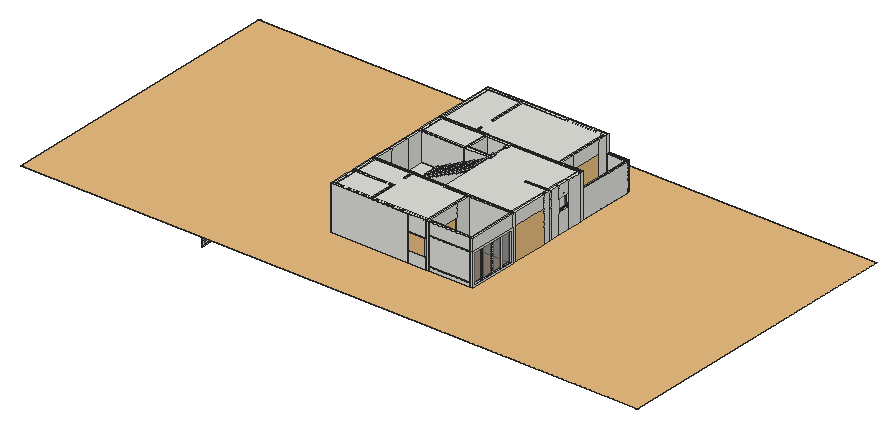
# SketchUp Ruby script. Lengths in inches.
U = 1.inch
M = Sketchup.active_model
def pt(a) = Geom::Point3d.new(a.map { |v| v * U })
def face(e, loops, mat)
  f = e.add_face(loops[0].map { |a| pt(a) })
  loops[1..].each { |l| e.add_face(l.map { |a| pt(a) }).erase! }
  f.material = f.back_material = mat if mat
  f
end
# faces: each face lists its corners as indices into pts; further lists are holes
def faces(e, pts, list, mat = nil) = list.each { |f| face(e, (f[0].is_a?(Array) ? f : [f]).map { |l| l.map { |i| pts[i] } }, mat) }
# xy, xz, yz: faces in a plane at the given z, y or x. An outline is a flat list of corners, or four numbers for a rectangle; further outlines are holes
def ring(l) = l.size == 4 ? [[l[0], l[1]], [l[2], l[1]], [l[2], l[3]], [l[0], l[3]]] : l.each_slice(2).to_a
def flat(e, list, mat, &to3) = list.each { |f| face(e, (f[0].is_a?(Array) ? f : [f]).map { |l| ring(l).map { |u, v| to3.(u, v) } }, mat) }
def xy(e, z, list, mat = nil) = flat(e, list, mat) { |x, y| [x, y, z] }
def xz(e, y, list, mat = nil) = flat(e, list, mat) { |x, z| [x, y, z] }
def yz(e, x, list, mat = nil) = flat(e, list, mat) { |y, z| [x, y, z] }
def lines(e, pts, list) = list.each { |a, b| e.add_line(pt(pts[a]), pt(pts[b])) }
# prism: a flat outline (further loops are holes) pulled along v
def prism(e, loops, v, mat = nil)
  f = face(e, loops, mat); d = Geom::Vector3d.new(v.map { |x| x * U })
  f.pushpull(f.normal.samedirection?(d) ? d.length : -d.length)
end
def box(e, o, s, mat = nil) = prism(e, [[o, [o[0] + s[0], o[1], o[2]], [o[0] + s[0], o[1] + s[1], o[2]], [o[0], o[1] + s[1], o[2]]]], [0, 0, s[2]], mat)
def at(x, y, z, deg = 0) = Geom::Transformation.translation(pt([x, y, z])) * Geom::Transformation.rotation(ORIGIN, Z_AXIS, deg.degrees)
def axes(o, x, y, z) = Geom::Transformation.new([*x, 0, *y, 0, *z, 0, *pt(o).to_a, 1])
def part(name) = M.definitions.add(name)
# library, detail: a bought-in or finely detailed component or shape, given as its bounding box
def library(name, o, s) = part(name).tap { |d| box(d.entities, o, s) }
def detail(e, o, s) = box(e.add_group.entities, o, s)
def put(e, d, t, mat = nil) = e.add_instance(d, t).tap { |i| i.material = mat if mat }
def group(e, t, mat = nil) = e.add_group.tap { |g| g.transformation = t; g.material = mat if mat }.entities
root = M.entities
M.materials.add("BeigeGloss_500x700").color = [214, 201, 185]
M.materials.add("MADEIRAS PORTAS MOD 4").color = [48, 37, 30]
M.materials.add("Metal_07").color = [114, 116, 119]
M.materials.add("Metal_Aluminum_Anodized").color = [200, 209, 218]
M.materials.add("Translucent_Glass_Gray").color = [198, 198, 198]
M.materials["Translucent_Glass_Gray"].alpha = 0.2
M.materials.add("[0136_Charcoal]1").color = [35, 35, 35]
M.materials.add("[Color_008]2").color = [30, 30, 30]
M.materials.add("[Translucent Glass Gray]").color = [128, 128, 128]
M.materials["[Translucent Glass Gray]"].alpha = 0.5
M.materials.add("[Translucent_Glass_Gray]").color = [128, 128, 128]
M.materials["[Translucent_Glass_Gray]"].alpha = 0.5
M.materials.add("aidan_hegarty_redux").color = [127, 127, 127]
M.materials["aidan_hegarty_redux"].alpha = 0
M.materials.add("door-silver").color = [161, 152, 147]
M.materials.add("wood _table").color = [169, 145, 123]
c1 = library("EAST VILLa 27.dwg",[0,0,0],[1841.08,888.15,0.01])
c2 = part("Untitled (3)")
g1 = group(c2.entities,at(-587.35,0.56,0))
g2 = group(g1,at(0,36.17,0))
g3 = group(g2,at(0,0,0))
xy(g3,0,[[0,-36.17,1118.43,-19.76]],"BeigeGloss_500x700")
xy(g3,7.07,[[6.51,-36.17,1111.93,-19.76]],"BeigeGloss_500x700")
xy(g3,448.65,[[6.51,-36.17,1111.93,-19.76]],"BeigeGloss_500x700")
xy(g3,455.72,[[0,-36.17,1118.43,-19.76]],"BeigeGloss_500x700")
xz(g3,-36.17,[[6.51,7.07,1111.93,448.65]])
xz(g3,-36.17,[[[0,0,1118.43,455.72],[6.51,7.07,1111.93,448.65]]],"BeigeGloss_500x700")
xz(g3,-19.76,[[[0,0,1118.43,455.72],[6.51,7.07,1111.93,448.65]]],"BeigeGloss_500x700")
yz(g3,0,[[-36.17,0,-19.76,455.72]],"BeigeGloss_500x700")
yz(g3,6.51,[[-36.17,7.07,-19.76,448.65]],"BeigeGloss_500x700")
yz(g3,1111.93,[[-36.17,7.07,-19.76,448.65]],"BeigeGloss_500x700")
yz(g3,1118.43,[[-36.17,0,-19.76,455.72]],"BeigeGloss_500x700")
c3 = part("Group\#69")
p = [[0,43.31,5.11],[2.95,43.31,0],[2.95,0,0],[0,0,5.11]]
faces(c3.entities,p,[[0,1,2,3]],"[Translucent_Glass_Gray]")
c4 = part("Vwntilation+window")
put(c4.entities,c3,at(43.48,1.97,32.29))
put(c4.entities,c3,at(43.48,1.97,26.38))
put(c4.entities,c3,at(43.48,1.97,20.48))
put(c4.entities,c3,at(43.48,1.97,14.57))
put(c4.entities,c3,at(43.48,1.97,8.67))
put(c4.entities,c3,at(43.48,1.97,2.76))
g4 = group(c4.entities,at(43.48,0,0))
prism(g4,[[[1.97,47.24,39.37],[1.97,0,39.37],[1.97,0,0],[1.97,47.24,0]],[[1.97,45.28,1.97],[1.97,1.97,1.97],[1.97,1.97,37.4],[1.97,45.28,37.4]]],[-1.97,0,0])
c5 = part("Window frame")
prism(c5.entities,[[[0,70.87,0],[0,0,0],[0,0,47.24],[0,70.87,47.24]],[[0,1.97,1.97],[0,68.9,1.97],[0,68.9,45.28],[0,1.97,45.28]]],[7.875,0,0])
c6 = part("Window sash \#3")
xy(c6.entities,0,[[0,0,3.9375,16.73]])
xy(c6.entities,0.98,[[0,0.98,1.77,15.75],[1.77,0.98,2.85,15.75],[2.85,0.98,3.9375,15.75]])
xy(c6.entities,42.32,[[0,0.98,1.77,15.75],[1.77,0.98,2.85,15.75],[2.85,0.98,3.9375,15.75]])
xy(c6.entities,43.31,[[0,0,3.9375,16.73]])
xz(c6.entities,0,[[0,0,3.9375,43.31]])
xz(c6.entities,0.98,[[0,0.98,1.77,42.32],[1.77,0.98,2.85,42.32],[2.85,0.98,3.9375,42.32]])
xz(c6.entities,15.75,[[0,0.98,1.77,42.32],[1.77,0.98,2.85,42.32],[2.85,0.98,3.9375,42.32]])
xz(c6.entities,16.73,[[0,0,3.9375,43.31]])
yz(c6.entities,0,[[[0,0,16.73,43.31],[0.98,0.98,15.75,42.32]]])
yz(c6.entities,1.77,[[0.98,0.98,15.75,42.32]],"[Translucent_Glass_Gray]")
yz(c6.entities,2.85,[[0.98,0.98,15.75,42.32]],"[Translucent_Glass_Gray]")
yz(c6.entities,3.9375,[[[0,0,16.73,43.31],[0.98,0.98,15.75,42.32]]])
c7 = part("simple+window")
p = [[0,68.9,1.97],[0,35.43,1.97]]
lines(c7.entities,p,[[0,1]])
put(c7.entities,c5,at(0,0,0))
put(c7.entities,c6,axes([1.14,52.17,1.97],[0.71,0,0],[0,1,0],[0,0,1]))
put(c7.entities,c6,axes([1.14,1.97,1.97],[0.71,0,0],[0,1,0],[0,0,1]))
put(c7.entities,c6,axes([3.9375,18.7,1.97],[0.71,0,0],[0,1,0],[0,0,1]))
put(c7.entities,c6,axes([3.9375,35.43,1.97],[0.71,0,0],[0,1,0],[0,0,1]))
c8 = part("Component\#104")
box(c8.entities,[-0.79,0,0],[1.58,2.36,0.2])
c9 = part("Door pull handle")
xy(c9.entities,-28.59,[[0.39,-0.79,0.19,-0.76,0,-0.68,-0.16,-0.56,-0.29,-0.39,-0.37,-0.2,-0.39,0,1.18,0,1.15,-0.2,1.08,-0.39,0.95,-0.56,0.79,-0.68,0.6,-0.76]])
xy(c9.entities,-13.39,[[-0.39,0,1.18,0.79]])
xy(c9.entities,-12.99,[[-0.39,0,1.18,0.79]])
xy(c9.entities,7.09,[[-0.39,0,1.18,0.79]])
xy(c9.entities,7.48,[[-0.39,0,1.18,0.79]])
xy(c9.entities,30.47,[[0.39,-0.79,0.6,-0.76,0.79,-0.68,0.95,-0.56,1.08,-0.39,1.15,-0.2,1.18,0,-0.39,0,-0.37,-0.2,-0.29,-0.39,-0.16,-0.56,0,-0.68,0.19,-0.76]])
xz(c9.entities,0,[[-0.39,-28.59,1.18,-13.39],[-0.39,-12.99,1.18,7.09],[-0.39,7.48,1.18,30.47]])
xz(c9.entities,0.79,[[-0.39,-13.39,1.18,-12.99],[-0.39,7.09,1.18,7.48]])
yz(c9.entities,-0.39,[[0,-13.39,0.79,-12.99],[0,7.09,0.79,7.48]])
yz(c9.entities,1.18,[[0,-13.39,0.79,-12.99],[0,7.09,0.79,7.48]])
p = [[0.19,-0.76,30.47],[0,-0.68,30.47],[0,-0.68,-28.59],[0.19,-0.76,-28.59],[0.39,-0.79,30.47],[0.39,-0.79,-28.59],
  [0.6,-0.76,30.47],[0.6,-0.76,-28.59],[0.79,-0.68,30.47],[0.79,-0.68,-28.59],[-0.16,-0.56,30.47],[-0.16,-0.56,-28.59],
  [0.95,-0.56,30.47],[0.95,-0.56,-28.59],[-0.29,-0.39,30.47],[-0.29,-0.39,-28.59],[1.08,-0.39,30.47],[1.08,-0.39,-28.59],
  [-0.37,-0.2,30.47],[-0.37,-0.2,-28.59],[1.15,-0.2,30.47],[1.15,-0.2,-28.59],[-0.39,0,30.47],[-0.39,0,7.48],
  [-0.39,0,7.09],[-0.39,0,-12.99],[-0.39,0,-13.39],[-0.39,0,-28.59],[1.18,0,30.47],[1.18,0,-28.59],
  [1.18,0,-13.39],[1.18,0,-12.99],[1.18,0,7.09],[1.18,0,7.48]]
faces(c9.entities,p,[[0,1,2,3],[4,0,3,5],[6,4,5,7],[8,6,7,9],[1,10,11,2],[12,8,9,13],[10,14,15,11],[16,12,13,17],
  [14,18,19,15],[20,16,17,21],[18,22,23,24,25,26,27,19],[28,20,21,29,30,31,32,33]])
put(c9.entities,c8,axes([4.72,0.79,-7.35],[1,0,0],[0,0,1],[0,-1,0]))
c10 = part("Door glazing insert")
xy(c10.entities,0,[[0.79,7.09,8.66,18.9]],"aidan_hegarty_redux")
xy(c10.entities,0.39,[[[-0.39,0.58,0.79,0.58,0.79,5.91,8.66,5.91,8.66,1.18,0.79,1.18,0.79,0.58,9.84,0.58,9.84,58.46,-0.39,58.46,-0.39,57.875,8.66,57.875,8.66,53.15,0.79,53.15,0.79,57.875,-0.39,57.875],[0.79,20.08,8.66,38.98],[0.79,40.16,8.66,51.97],[0.79,7.09,8.66,18.9]]])
xy(c10.entities,0.39,[[0.79,1.18,8.66,5.91],[0.79,20.08,8.66,38.98],[0.79,40.16,8.66,51.97],[0.79,53.15,8.66,57.875]],"[Translucent Glass Gray]")
xz(c10.entities,1.18,[[0.79,0,8.66,0.39]])
xz(c10.entities,5.91,[[0.79,0,8.66,0.39]])
xz(c10.entities,7.09,[[0.79,0,8.66,0.39]])
xz(c10.entities,18.9,[[0.79,0,8.66,0.39]])
xz(c10.entities,20.08,[[0.79,0,8.66,0.39]])
xz(c10.entities,38.98,[[0.79,0,8.66,0.39]])
xz(c10.entities,40.16,[[0.79,0,8.66,0.39]])
xz(c10.entities,51.97,[[0.79,0,8.66,0.39]])
xz(c10.entities,53.15,[[0.79,0,8.66,0.39]])
xz(c10.entities,57.875,[[0.79,0,8.66,0.39]])
yz(c10.entities,-0.39,[[0,0,0.06,0.11,0.13,0.21,0.23,0.29,0.33,0.34,0.45,0.38,0.58,0.39,58.46,0.39,58.34,0.38,58.22,0.35,58.11,0.29,58.01,0.21,57.93,0.11,57.875,0],[57.875,0,57.93,0.11,58.01,0.21,58.11,0.29,58.22,0.35,58.34,0.38,58.46,0.39,58.59,0.38,58.71,0.35,58.82,0.29,58.92,0.21,59,0.11,59.06,0]])
yz(c10.entities,0.79,[[1.18,0,5.91,0.39],[7.09,0,18.9,0.39],[20.08,0,38.98,0.39],[40.16,0,51.97,0.39],[53.15,0,57.875,0.39]])
yz(c10.entities,8.66,[[1.18,0,5.91,0.39],[5.91,0,7.09,0.39],[7.09,0,18.9,0.39],[18.9,0,20.08,0.39],[20.08,0,38.98,0.39],
  [38.98,0,40.16,0.39],[40.16,0,51.97,0.39],[51.97,0,53.15,0.39],[53.15,0,57.875,0.39]])
yz(c10.entities,9.84,[[0,0,59.06,0,59,0.11,58.92,0.21,58.82,0.29,58.71,0.35,58.59,0.38,58.46,0.39,0.58,0.39,0.45,0.38,0.33,0.34,0.23,0.29,0.13,0.21,0.06,0.11]])
p = [[-0.39,0.06,0.11],[-0.39,0,0],[0.79,0,0],[9.84,0,0],[9.84,0.06,0.11],[-0.39,59.06,0],
  [-0.39,59,0.11],[9.84,59,0.11],[9.84,59.06,0],[-0.39,0.13,0.21],[9.84,0.13,0.21],[-0.39,58.92,0.21],
  [9.84,58.92,0.21],[-0.39,0.23,0.29],[9.84,0.23,0.29],[-0.39,58.82,0.29],[9.84,58.82,0.29],[-0.39,0.33,0.34],
  [9.84,0.33,0.34],[-0.39,0.45,0.38],[9.84,0.45,0.38],[-0.39,58.71,0.35],[-0.39,58.59,0.38],[9.84,58.59,0.38],
  [9.84,58.71,0.35],[-0.39,0.58,0.39],[9.84,0.58,0.39],[0.79,0.58,0.39],[-0.39,58.46,0.39],[9.84,58.46,0.39]]
faces(c10.entities,p,[[0,1,2,3,4],[5,6,7,8],[9,0,4,10],[6,11,12,7],[13,9,10,14],[11,15,16,12],[17,13,14,18],[19,17,18,20],
  [21,22,23,24],[15,21,24,16],[25,19,20,26,27],[22,28,29,23]])
lines(c10.entities,p,[[27,2]])
c11 = part("dvere")
xy(c11.entities,0,[[0,-0.2,39.37,1.18]],"MADEIRAS PORTAS MOD 4")
xy(c11.entities,3.9375,[[0,-0.2,39.37,0]],"MADEIRAS PORTAS MOD 4")
xy(c11.entities,11.8125,[[14.96,0,24.41,1.18]],"MADEIRAS PORTAS MOD 4")
xy(c11.entities,70.87,[[14.96,0,24.41,1.18]],"MADEIRAS PORTAS MOD 4")
xy(c11.entities,76.77,[[0,-0.2,39.37,0]],"MADEIRAS PORTAS MOD 4")
xy(c11.entities,78.74,[[0,-0.2,39.37,1.18]],"MADEIRAS PORTAS MOD 4")
xz(c11.entities,-0.2,[[0,0,39.37,3.9375],[0,76.77,39.37,78.74]],"MADEIRAS PORTAS MOD 4")
xz(c11.entities,0,[[[0,3.9375,39.37,76.77],[14.96,11.8125,24.41,70.87]]],"MADEIRAS PORTAS MOD 4")
xz(c11.entities,1.18,[[[0,0,39.37,78.74],[14.96,11.8125,24.41,70.87]]],"MADEIRAS PORTAS MOD 4")
yz(c11.entities,0,[[-0.2,0,-0.2,3.9375,0,3.9375,0,76.77,-0.2,76.77,-0.2,78.74,1.18,78.74,1.18,0]],"MADEIRAS PORTAS MOD 4")
yz(c11.entities,14.96,[[0,11.8125,1.18,70.87]],"MADEIRAS PORTAS MOD 4")
yz(c11.entities,24.41,[[0,11.8125,1.18,70.87]],"MADEIRAS PORTAS MOD 4")
yz(c11.entities,39.37,[[-0.2,0,1.18,0,1.18,78.74,-0.2,78.74,-0.2,77.76,0,76.77,0,3.9375,-0.2,3.9375],[-0.2,76.77,0,76.77,-0.2,77.76]],"MADEIRAS PORTAS MOD 4")
p = [[19.69,0,70.87],[19.69,1.18,78.74],[33.46,0,27.01],[33.46,0,25.4375],[24.41,0,69.69],[23.62,0,69.69],
  [23.62,1.19,69.69]]
lines(c11.entities,p,[[0,1],[2,3],[4,5],[5,6]])
put(c11.entities,c9,at(33.86,-0.79,40.4),"Metal_07")
put(c11.entities,c10,axes([24.41,1.19,11.8125],[-1,0,0],[0,0,1],[0,1,0]),"wood _table")
put(c11.entities,c10,axes([14.96,0,11.8125],[1,0,0],[0,0,1],[0,-1,0]),"MADEIRAS PORTAS MOD 4")
c12 = part("Glazed entrance door \#1")
put(c12.entities,c11,at(80.69,2.95,0),"MADEIRAS PORTAS MOD 4")
c13 = part("Glazed entrance door")
put(c13.entities,c12,at(-80.69,-2.76,0),"MADEIRAS PORTAS MOD 4")
c14 = library("30inch+Toilet+door",[0,0,0],[5.5,37.8,85])
c15 = library("AS-120-mm\#1",[0,0,0],[106.47,4.72,96])
c16 = part("Grupo\#90")
xy(c16.entities,0,[[0,0,0.79,0.79]],"[Color_008]2")
xy(c16.entities,0.79,[[0,0,0.79,0.79]],"[Color_008]2")
xz(c16.entities,0,[[0,0,0.79,0.79],[-3.9375,0.79,-3.62,0.91,-3.3,1,-2.97,1.08,-2.64,1.14,-2.31,1.17,-1.97,1.18,-1.63,1.17,-1.3,1.14,-0.96,1.08,-0.64,1,-0.31,0.91,0,0.79,0.79,0.79,0.4375,1.02,0.0625,1.22,-0.33,1.37,-0.74,1.48,-1.15,1.55,-1.57,1.57,-2,1.55,-2.41,1.48,-2.82,1.37,-3.21,1.22,-3.59,1.02]],"[Color_008]2")
xz(c16.entities,0.79,[[0,0,0.79,0.79],[-3.9375,0.79,-3.59,1.02,-3.21,1.22,-2.82,1.37,-2.41,1.48,-2,1.55,-1.57,1.57,-1.15,1.55,-0.74,1.48,-0.33,1.37,0.0625,1.22,0.4375,1.02,0.79,0.79,0,0.79,-0.31,0.91,-0.64,1,-0.96,1.08,-1.3,1.14,-1.63,1.17,-1.97,1.18,-2.31,1.17,-2.64,1.14,-2.97,1.08,-3.3,1,-3.62,0.91]],"[Color_008]2")
yz(c16.entities,0,[[0,0,0.79,0.79]],"[Color_008]2")
yz(c16.entities,0.79,[[0,0,0.79,0.79]],"[Color_008]2")
p = [[-3.9375,0,0.79],[-3.59,0,1.02],[-3.59,0.79,1.02],[-3.9375,0.79,0.79],[-3.62,0,0.91],[-3.62,0.79,0.91],
  [0,0,0.79],[-0.31,0,0.91],[-0.31,0.79,0.91],[0,0.79,0.79],[0.4375,0,1.02],[0.79,0,0.79],
  [0.79,0.79,0.79],[0.4375,0.79,1.02],[-3.3,0,1],[-3.3,0.79,1],[-0.64,0,1],[-0.64,0.79,1],
  [-3.21,0,1.22],[-3.21,0.79,1.22],[-2.97,0,1.08],[-2.97,0.79,1.08],[-0.96,0,1.08],[-0.96,0.79,1.08],
  [0.0625,0,1.22],[0.0625,0.79,1.22],[-2.64,0,1.14],[-2.64,0.79,1.14],[-2.31,0,1.17],[-2.31,0.79,1.17],
  [-1.3,0,1.14],[-1.63,0,1.17],[-1.63,0.79,1.17],[-1.3,0.79,1.14],[-2.82,0,1.37],[-2.82,0.79,1.37],
  [-1.97,0,1.18],[-1.97,0.79,1.18],[-0.33,0,1.37],[-0.33,0.79,1.37],[-2.41,0,1.48],[-2.41,0.79,1.48],
  [-0.74,0,1.48],[-0.74,0.79,1.48],[-2,0,1.55],[-2,0.79,1.55],[-1.15,0,1.55],[-1.15,0.79,1.55],
  [-1.57,0,1.57],[-1.57,0.79,1.57]]
faces(c16.entities,p,[[0,1,2,3],[4,0,3,5],[6,7,8,9],[10,11,12,13],[14,4,5,15],[7,16,17,8],[1,18,19,2],[20,14,15,21],
  [16,22,23,17],[24,10,13,25],[26,20,21,27],[28,26,27,29],[30,31,32,33],[22,30,33,23],[18,34,35,19],[36,28,29,37],
  [31,36,37,32],[38,24,25,39],[34,40,41,35],[42,38,39,43],[40,44,45,41],[46,42,43,47],[44,48,49,45],[48,46,47,49]],"[Color_008]2")
c17 = part("Awning window")
xy(c17.entities,0,[[0,0,39.37,1.57]],"[0136_Charcoal]1")
xy(c17.entities,0.79,[[0.79,0,38.58,1.57]],"[0136_Charcoal]1")
xy(c17.entities,30.71,[[0.79,0,38.58,1.57]],"[0136_Charcoal]1")
xy(c17.entities,31.5,[[0,0,39.37,1.57]],"[0136_Charcoal]1")
xz(c17.entities,0,[[[0,0,39.37,31.5],[0.79,0.79,38.58,30.71]]],"[0136_Charcoal]1")
xz(c17.entities,1.57,[[[0,0,39.37,31.5],[0.79,0.79,38.58,30.71]]],"[0136_Charcoal]1")
yz(c17.entities,0,[[0,0,1.57,31.5]],"[0136_Charcoal]1")
yz(c17.entities,0.79,[[0,0.79,1.57,0.79,1.57,17.41,0.78,17.0625,0.49,17.72,1.57,18.2,1.57,30.71,0,30.71],[0.78,17.0625,0.49,17.72,1.57,18.2,1.57,17.41],[1.57,17.41,1.57,18.2,6.39,20.3,6.73,20.5,7.1,19.87,6.75,19.67]],"[0136_Charcoal]1")
yz(c17.entities,1.18,[[15.57,4.4,6.75,19.67,7.1,19.87,6.73,20.5,6.39,20.3,0.61,30.31,1.29,30.71,16.25,4.8],[0.78,17.0625,6.75,19.67,6.39,20.3,0.49,17.72],[6.75,19.67,7.1,19.87,6.73,20.5,6.39,20.3]],"[0136_Charcoal]1")
yz(c17.entities,1.97,[[15.35,5.18,1.17,29.73,1.52,29.93,15.6875,5.38]],"Translucent_Glass_Gray")
yz(c17.entities,1.97,[[15.18,5.08,15.35,5.18,1.17,29.73,1,29.63],[15.6875,5.38,15.86,5.48,1.6875,30.03,1.52,29.93]],"[0136_Charcoal]1")
yz(c17.entities,37.4,[[15.35,5.18,15.6875,5.38,1.52,29.93,1.17,29.73]],"Translucent_Glass_Gray")
yz(c17.entities,37.4,[[15.18,5.08,1,29.63,1.17,29.73,15.35,5.18],[15.6875,5.38,1.52,29.93,1.6875,30.03,15.86,5.48]],"[0136_Charcoal]1")
yz(c17.entities,38.1875,[[15.57,4.4,16.25,4.8,1.29,30.71,0.61,30.31,6.39,20.3,6.73,20.5,7.1,19.87,6.75,19.67],[0.78,17.0625,0.49,17.72,6.39,20.3,6.75,19.67],[6.75,19.67,6.39,20.3,6.73,20.5,7.1,19.87]],"[0136_Charcoal]1")
yz(c17.entities,38.58,[[0,0.79,0,30.71,1.57,30.71,1.57,18.2,0.49,17.72,0.78,17.0625,1.57,17.41,1.57,0.79],[0.78,17.0625,1.57,17.41,1.57,18.2,0.49,17.72],[1.57,17.41,6.75,19.67,7.1,19.87,6.73,20.5,6.39,20.3,1.57,18.2]],"[0136_Charcoal]1")
yz(c17.entities,39.37,[[0,0,1.57,31.5]],"[0136_Charcoal]1")
p = [[1.18,0.61,30.31],[1.18,6.39,20.3],[1.18,6.75,19.67],[1.18,15.57,4.4],[38.1875,15.57,4.4],[38.1875,6.75,19.67],
  [38.1875,6.39,20.3],[38.1875,0.61,30.31],[37.4,15.18,5.08],[1.97,15.18,5.08],[1.97,1,29.63],[37.4,1,29.63],
  [1.18,16.25,4.8],[38.1875,16.25,4.8],[1.18,1.29,30.71],[38.1875,1.29,30.71],[37.4,15.86,5.48],[37.4,1.6875,30.03],
  [1.97,1.6875,30.03],[1.97,15.86,5.48],[37.4,15.35,5.18],[1.97,15.35,5.18],[37.4,1.17,29.73],[1.97,1.17,29.73],
  [1.97,15.6875,5.38],[37.4,15.6875,5.38],[1.97,1.52,29.93],[37.4,1.52,29.93],[1.18,0.78,17.0625],[1.18,0.49,17.72],
  [0.79,0.49,17.72],[0.79,0.78,17.0625],[38.58,0.78,17.0625],[38.58,0.49,17.72],[38.1875,0.49,17.72],[38.1875,0.78,17.0625],
  [0.79,1.57,17.41],[0.79,6.75,19.67],[38.58,6.75,19.67],[38.58,1.57,17.41],[0.79,6.39,20.3],[0.79,1.57,18.2],
  [38.58,1.57,18.2],[38.58,6.39,20.3],[0.79,7.1,19.87],[1.18,7.1,19.87],[38.1875,7.1,19.87],[38.58,7.1,19.87],
  [0.79,6.73,20.5],[1.18,6.73,20.5],[38.1875,6.73,20.5],[38.58,6.73,20.5]]
faces(c17.entities,p,[[[0,1,2,3,4,5,6,7],[8,9,10,11]],[12,13,4,3],[[14,15,13,12],[16,17,18,19]],[8,20,21,9],[19,24,25,16],[28,29,30,31],[32,33,34,35],[28,31,36,37,2],
  [32,35,5,38,39],[40,41,30,29,1],[6,34,33,42,43],[2,37,44,45],[38,5,46,47],[44,48,49,45],[46,50,51,47],[40,1,49,48],
  [6,43,51,50],[10,23,22,11],[17,27,26,18],[15,14,0,7]],"[0136_Charcoal]1")
faces(c17.entities,p,[[21,20,22,23],[24,25,20,21],[25,24,26,27],[27,26,23,22]],"Translucent_Glass_Gray")
put(c17.entities,c16,axes([21.2,15.57,4.4],[0.93,0,0],[0,-0.5,0.86603],[0,-0.86603,-0.5]))
c18 = part("Untitled\#1")
put(c18.entities,c17,axes([31.92,9,0],[-0.81077,0,0],[0,-0.55376,0],[0,0,1.143]))
c19 = part("Untitled (4)")
put(c19.entities,c18,at(0,0,0))
c20 = library("Untitled (1)",[64.55,2.64,0],[5.19,55.84,46.48])
c21 = library("AS-120-mm\#2",[0,0,0],[96.73,4.72,96])
c22 = library("AS-120-mm\#3",[0,0,0],[97.15,4.72,96])
c23 = library("AS-120-mm\#4",[0,0,0],[84.45,4.72,96])
c24 = part("Group\#63")
box(c24.entities,[0,0,0],[12.06,48.26,6])
c25 = part("Door panel")
xy(c25.entities,0.39,[[6.02,0,23.62,1.25]],"door-silver")
xy(c25.entities,84,[[6.02,0,23.62,1.25]],"door-silver")
xz(c25.entities,0,[[6.02,0.39,23.62,84]],"door-silver")
xz(c25.entities,1.25,[[6.02,0.39,23.62,84]],"door-silver")
yz(c25.entities,6.02,[[0,0.39,1.25,84]])
yz(c25.entities,23.62,[[0,0.39,1.25,84]],"door-silver")
c26 = part("Door3")
put(c26.entities,c25,at(9.9375,0,0))
put(c26.entities,c25,axes([21.75,0,0],[-1,0,0],[0,1,0],[0,0,1]))
c27 = part("Vertical post")
prism(c27.entities,[[[5.91,11.16,0.39],[5.91,3.9375,0.39],[1.97,0,0.39],[-1.97,0,0.39],[-1.97,11.16,0.39]]],[0,0,82.28])
c28 = part("ske11")
put(c28.entities,c26,axes([1.25,0,-9.5],[1,0,0],[0,0,-1],[0,1,0]))
put(c28.entities,c27,axes([-6.53,0,0.8],[1,0,0],[0,0,-1],[0,1,0]))
put(c28.entities,c27,axes([40.72,0,0.8],[-1,0,0],[0,0,-1],[0,1,0]))
g5 = group(c28.entities,at(-5.875,0.79,-9.5))
xy(g5,10.3,[[-2.62,81.89,48.56,107.875]])
xz(g5,81.89,[[-2.62,0,48.56,10.3]])
xz(g5,107.875,[[-2.62,9.5,48.56,10.3]])
yz(g5,-2.62,[[81.89,9.5,107.875,10.3]])
yz(g5,48.56,[[81.89,9.5,107.875,10.3]])
c29 = part("3\#1")
prism(c29.entities,[[[0.52,2.78,0],[2.34,3,0],[2.5,2.38,0],[2.81,1.93,0],[3.23,1.65,0],[3.74,1.5625,0],[4.27,1.67,0],[4.72,2.01,0],[5.02,2.53,0],[5.12,3.2,0],[5.02,3.84,0],[4.74,4.33,0],[4.3125,4.64,0],[3.8,4.74,0],[2.9375,4.6,0],[3.15,6.14,0],[3.82,6.21,0],[4.3125,6.47,0],[4.61,6.88,0],[4.71,7.4,0],[4.64,7.85,0],[4.42,8.2,0],[4.08,8.42,0],[3.64,8.49,0],[3.1875,8.41,0],[2.81,8.16,0],[2.54,7.74,0],[2.39,7.18,0],[0.66,7.47,0],[0.88,8.27,0],[1.2,8.9,0],[1.64,9.37,0],[2.22,9.74,0],[2.92,9.96,0],[3.6875,10.04,0],[4.35,9.98,0],[4.94,9.82,0],[5.46,9.54,0],[5.92,9.15,0],[6.22,8.78,0],[6.43,8.38,0],[6.5625,7.96,0],[6.61,7.52,0],[6.52,6.9,0],[6.25,6.35,0],[5.81,5.87,0],[5.19,5.45,0],[5.95,5.16,0],[6.54,4.64,0],[6.92,3.95,0],[7.05,3.12,0],[6.99,2.5,0],[6.8125,1.92,0],[6.52,1.39,0],[6.1,0.91,0],[5.6,0.51,0],[5.04,0.23,0],[4.42,0.06,0],[3.75,0,0],[3.11,0.05,0],[2.53,0.19,0],[2,0.43,0],[1.54,0.77,0],[1.14,1.18,0],[0.84,1.65,0],[0.63,2.1875,0]]],[0,0,0.98])
xy(root,0,[[364.61,22.01,787.73,433.49],[364.61,433.49,725.93,606.85]])
xy(root,132,[[374.77,22.01,657.98,22.01,657.98,171.45,581.36,171.45,581.36,175.89,374.77,175.89],[581.36,171.45,657.98,175.89],[657.98,171.45,787.73,175.89],[581.36,175.89,787.73,424.6],[365.67,347.77,504.375,433.49],
  [365.67,433.49,725.93,606.85]])
p = [[726.35,473.5,0],[725.93,473.5,0],[725.93,569.17,0],[726.35,569.17,0],[365.67,175.89,132],[365.67,347.77,132],
  [787.73,433.49,132],[787.73,424.6,132],[725.93,433.49,132],[374.77,175.89,132]]
lines(root,p,[[0,1],[2,3],[4,5],[6,7],[8,6],[9,4]])
put(root,c1,at(-395.06,-183.9375,0))
put(root,c2,axes([721.38,21.82,12],[0.10949,0,0],[0,0.3472,0],[0,0,0.18409]))
put(root,c4,at(-43.48,0,-155.89))
put(root,c7,axes([781.41,22.01,0],[0.84272,0,0],[0,2.10872,0],[0,0,2.032]))
put(root,c13,axes([686.56,425.97,0],[-1.06989,0,0],[0,1,0],[0,0,1.2192]))
put(root,c14,axes([409.27,103.5,0],[0,1,0],[0.80075,0,0],[0,0,1.12941]))
put(root,c14,axes([416.68,422.91,0],[0,1,0],[0.80075,0,0],[0,0,1.12941]))
put(root,c15,at(787.73,180.34,0,90))
put(root,c19,at(787.73,344.59,60,90))
put(root,c20,axes([651.65,-44.99,35.92],[0,1,0],[-0.95,0,0],[0,0,1.03451]))
put(root,c21,at(650.97,30.9,0,90))
put(root,c22,at(725.93,473.5,0,90))
put(root,c23,at(688.25,606.85,0,-180))
put(root,c4,axes([413.1875,74.93,60],[-1,0,0],[0,0.51075,0],[0,0,0.93]))
put(root,c4,axes([413.1875,361.1,60],[-1,0,0],[0,0.51075,0],[0,0,0.93]))
put(root,c2,axes([758.08,600.96,0],[0.05475,0,0],[0,0.3472,0],[0,0,0.18409]))
put(root,c2,axes([787.93,521.6,0],[0,0.15001,0],[-0.3472,0,0],[0,0,0.18409]))
g6 = group(root,at(688.25,569.17,0))
xy(g6,0,[[28.57,1.48,37.68,28.57],[0,28.57,37.68,37.68]])
xy(g6,132,[[28.57,1.48,37.68,28.57],[0,28.57,37.68,37.68]])
xz(g6,1.48,[[28.57,0,37.68,132]])
xz(g6,28.57,[[0,0,28.57,132],[28.57,0,37.68,132]])
xz(g6,37.68,[[0,0,37.68,132]])
yz(g6,0,[[28.57,0,37.68,132]])
yz(g6,28.57,[[1.48,0,28.57,132]])
yz(g6,37.68,[[1.48,0,28.57,132],[28.57,0,37.68,132]])
p = [[37.68,1.48,0],[37.68,0,0],[28.57,0,0],[28.57,1.48,0]]
lines(g6,p,[[0,1],[2,1],[2,3]])
g7 = group(root,at(603.8,597.75,0))
box(g7,[0,0,96],[84.45,9.1,36])
g8 = group(root,at(364.61,22.01,0))
prism(g8,[[[0,8.89,0],[1.06,8.89,0],[10.16,8.89,0],[117.05,8.89,0],[121.5,8.89,0],[231.5625,8.89,0],[231.5625,0,0],[0,0,0]]],[0,0,132])
g9 = group(root,at(365.67,30.9,0))
box(g9,[0,0,0],[9.1,44.03,132])
g10 = group(root,at(596.18,22.01,0))
box(g10,[0,0,0],[52.7,8.89,36])
box(g10,[0,0,84],[52.7,8.89,48])
p = [[0,8.89,36],[0,8.89,84],[52.7,8.89,36],[52.7,8.89,84]]
lines(g10,p,[[0,1],[2,3]])
g11 = group(root,at(648.88,22.01,0))
prism(g11,[[[0,8.89,0],[9.1,8.89,0],[9.1,6.98,0],[9.1,0,0],[0,0,0]]],[0,0,132])
g12 = group(root,at(365.67,99.06,0))
box(g12,[0,0,0],[9.1,4.44,132])
g13 = group(root,at(365.67,103.5,0))
prism(g13,[[[0,0,0],[0,6.14,0],[9.1,6.14,0],[43.6,6.14,0],[43.6,0,0],[9.1,0,0]]],[0,0,132])
g14 = group(root,at(365.67,109.64,0))
box(g14,[0,0,0],[9.1,66.25,132])
g15 = group(root,at(365.67,175.89,0))
prism(g15,[[[0,0,0],[0,4.44,0],[9.1,4.44,0],[236.64,4.44,0],[236.64,0,0],[120.4375,0,0],[115.99,0,0],[9.1,0,0]]],[0,0,132])
g16 = group(root,at(481.66,30.9,0))
box(g16,[0,0,0],[4.44,72.6,132])
g17 = group(root,at(439.54,103.5,0))
prism(g17,[[[42.12,0,0],[0,0,0],[0,6.14,0],[46.57,6.14,0],[46.57,0,0]]],[0,0,132])
g18 = group(root,at(481.66,148.59,0))
box(g18,[0,0,0],[4.44,27.3,132])
g19 = group(root,at(648.88,127.63,0))
box(g19,[0,0,0],[9.1,43.81,132])
g20 = group(root,at(778.63,286.81,0))
box(g20,[0,0,0],[9.1,23.28,132])
g21 = group(root,at(778.63,314.54,0))
box(g21,[0,0,0],[9.1,30.06,132])
g22 = group(root,at(713.86,310.09,0))
prism(g22,[[[73.87,4.44,0],[73.87,0,0],[64.77,0,0],[0,0,0],[0,4.44,0],[64.77,4.44,0]]],[0,0,132])
g23 = group(root,at(778.63,380.79,0))
box(g23,[0,0,0],[9.1,43.81,132])
g24 = group(root,at(716.83,424.81,0))
prism(g24,[[[0,8.68,0],[9.1,8.68,0],[70.91,8.68,0],[70.91,0,0],[0,0,0],[0,4.23,0]]],[0,0,132])
g25 = group(root,at(716.83,433.49,0))
box(g25,[0,0,0],[9.1,40,132])
g26 = group(root,at(716.83,473.5,0))
xy(g26,96,[[0,0,9.1,97.15]])
xy(g26,132,[[0,0,9.1,97.15]])
xz(g26,0,[[0,96,9.1,132]])
xz(g26,97.15,[[0,96,9.1,132]])
yz(g26,0,[[95.67,0,97.15,96],[0,96,95.67,132],[95.67,96,97.15,132]])
yz(g26,9.1,[[0,96,97.15,132]])
p = [[0,0,0],[0,0,96],[0,95.67,0]]
lines(g26,p,[[0,1],[0,2]])
g27 = group(root,at(686.56,424.6,0))
prism(g27,[[[0,4.44,0],[30.27,4.44,0],[30.27,0.21,0],[30.27,0,0],[0,0,0]]],[0,0,132])
g28 = group(root,at(581.36,424.6,0))
box(g28,[0,0,0],[63.08,4.44,132])
g29 = group(root,at(365.67,347.77,0))
prism(g29,[[[0,4.44,0],[9.1,4.44,0],[137.37,4.44,0],[137.37,0,0],[9.1,0,0],[0,0,0]]],[0,0,132])
g30 = group(root,at(446.95,424.6,0))
prism(g30,[[[28.79,4.44,0],[56.09,4.44,0],[56.09,0,0],[0,0,0],[0,4.44,0],[24.13,4.44,0]]],[0,0,132])
g31 = group(root,at(365.67,424.6,0))
prism(g31,[[[0,0,0],[0,4.44,0],[9.1,4.44,0],[51.22,4.44,0],[51.22,0,0],[9.1,0,0]]],[0,0,132])
g32 = group(root,at(471.08,429.05,0))
box(g32,[0,0,0],[4.66,18.41,132])
g33 = group(root,at(471.08,489.8,0))
box(g33,[0,0,0],[4.66,107.95,132])
g34 = group(root,at(644.44,171.45,0))
xy(g34,0,[[4.44,0,143.3,4.44],[0,4.44,4.44,8.89],[4.44,4.44,143.3,8.89]])
xy(g34,132,[[4.44,0,143.3,0,143.3,8.89,0,8.89,0,4.44,4.44,4.44]])
xz(g34,0,[[4.44,0,143.3,132]])
xz(g34,4.44,[[0,0,4.44,132]])
xz(g34,8.89,[[0,0,4.44,132],[4.44,0,143.3,132]])
yz(g34,0,[[4.44,0,8.89,132]])
yz(g34,4.44,[[0,0,4.44,132]])
yz(g34,143.3,[[0,0,8.89,132]])
g35 = group(root,at(365.67,597.75,0))
prism(g35,[[[0,9.1,0],[238.125,9.1,0],[238.125,0,0],[110.07,0,0],[105.41,0,0],[9.1,0,0],[0,0,0]]],[0,0,132])
g36 = group(root,at(365.67,429.05,0))
box(g36,[0,0,0],[9.1,168.7,132])
g37 = group(root,at(365.67,385.23,0))
box(g37,[0,0,0],[9.1,39.37,132])
g38 = group(root,at(365.67,352.21,0))
box(g38,[0,0,0],[9.1,8.89,132])
g39 = group(root,at(503.04,347.77,0))
g40 = group(g39,at(69.21,8.89,0))
box(g40,[0,0,0],[9.1,12.06,132])
g41 = group(g39,at(69.21,60.11,0))
box(g41,[0,0,0],[9.1,12.06,132])
g42 = group(g39,at(0,72.18,0))
prism(g42,[[[8.89,0,0],[0,0,0],[0,4.66,0],[0,9.1,0],[78.32,9.1,0],[78.32,4.66,0],[78.32,0,0],[69.21,0,0]]],[0,0,132])
g43 = group(g39,at(0,0,0))
prism(g43,[[[78.32,0,0],[0,0,0],[0,4.44,0],[0,8.89,0],[8.89,8.89,0],[69.21,8.89,0],[78.32,8.89,0]]],[0,0,132])
g44 = group(g39,at(0,8.89,0))
box(g44,[0,0,0],[8.89,63.29,132])
g45 = group(root,at(644.44,424.6,0))
box(g45,[0,0,96],[42.12,4.44,36])
g46 = group(root,at(416.89,424.6,0))
box(g46,[0,0,96],[30.06,4.44,36])
g47 = group(root,at(409.27,103.5,0))
box(g47,[0,0,96],[30.27,6.14,36])
g48 = group(root,at(657.98,22.01,0))
box(g48,[0,0,96],[129.75,6.98,36])
g49 = group(root,at(422.82,180.34,0))
xy(g49,0,[[0,0,12.06,48.26]])
g50 = group(root,at(374.77,180.34,0))
box(g50,[0,0,0],[48.05,48.47,6])
g51 = group(root,at(374.77,287.44,36))
box(g51,[0,0,0],[48.05,12.06,6])
g52 = group(root,at(374.77,228.8125,6))
box(g52,[0,0,0],[48.05,11.43,6])
g53 = group(root,at(374.77,240.24,12))
box(g53,[0,0,0],[48.05,12.06,6])
g54 = group(root,at(374.77,252.31,18))
box(g54,[0,0,0],[48.05,11.43,6])
g55 = group(root,at(374.77,263.74,24))
box(g55,[0,0,0],[48.05,11.64,6])
g56 = group(root,at(374.77,275.38,30))
box(g56,[0,0,0],[48.05,12.06,6])
g57 = group(root,at(374.77,299.51,42))
box(g57,[0,0,0],[48.05,48.26,6])
put(root,c24,at(422.82,299.51,48))
put(root,c24,at(434.89,299.51,54))
put(root,c24,at(446.95,299.51,60))
put(root,c24,at(459.02,299.51,66))
put(root,c24,at(471.08,299.51,72))
put(root,c24,at(483.15,299.51,78))
put(root,c24,at(495.21,299.51,84))
put(root,c24,at(507.28,299.51,90))
put(root,c24,at(519.34,299.51,96))
put(root,c24,at(531.41,299.51,102))
put(root,c24,at(543.47,299.51,108))
put(root,c24,at(555.54,299.51,114))
put(root,c24,at(567.6,299.51,120))
g58 = group(root,at(365.67,74.93,0))
box(g58,[0,0,0],[9.1,24.13,60])
box(g58,[0,0,96],[9.1,24.13,36])
p = [[9.1,24.13,60],[9.1,24.13,96],[9.1,0,60],[9.1,0,96]]
lines(g58,p,[[0,1],[2,3]])
g59 = group(root,at(365.67,298.875,0))
box(g59,[0,0,0],[9.1,48.89,132])
g60 = group(root,at(365.67,180.34,0))
box(g60,[0,0,0],[9.1,58.42,132])
g61 = group(root,at(365.67,238.76,0))
box(g61,[0,0,0],[9.1,60.11,132])
g62 = group(root,at(365.67,361.1,0))
box(g62,[0,0,0],[9.1,24.13,60])
box(g62,[0,0,96],[9.1,24.13,36])
p = [[9.1,24.13,60],[9.1,24.13,96],[9.1,0,60],[9.1,0,96]]
lines(g62,p,[[0,1],[2,3]])
g63 = group(root,at(778.63,344.59,0))
box(g63,[0,0,0],[9.1,36.19,60])
box(g63,[0,0,96],[9.1,36.19,36])
p = [[0,0,60],[0,0,96],[0,36.19,60],[0,36.19,96]]
lines(g63,p,[[0,1],[2,3]])
g64 = group(root,at(778.63,180.34,0))
box(g64,[0,0,96],[9.1,106.47,36])
g65 = group(root,at(780.54,22.01,0))
prism(g65,[[[7.2,149.4375,96],[7.2,0,96],[0,0,96],[0,6.98,96],[0,149.4375,96]]],[0,0,36])
p = [[0,0,0],[0,149.4375,0]]
lines(g65,p,[[0,1]])
g66 = group(root,at(648.88,30.9,0))
box(g66,[0,0,96],[9.1,96.73,36])
g67 = group(root,at(602.3125,175.88,0))
put(g67,c13,axes([42.12,1.78,0],[-1.06989,0,0],[0,-1,0],[0,0,1.2192]))
g68 = group(g67,at(0,0.02,0))
box(g68,[0,0,96],[42.12,4.44,36])
g69 = group(root,at(657.98,22.01,0))
box(g69,[0,0,0],[122.55,6.98,12])
g70 = group(root,at(581.36,347.77,0))
g71 = group(g70,at(-0.87,0,0))
g72 = group(g71,at(-0.52,81.05,0))
prism(g72,[[[0.52,-0.35,108.27],[0.52,-0.35,3.9375],[0.52,0.23,3.9375],[0.52,0.23,23.52],[0.52,0.09,23.52],[0.52,0.09,23.72],[0.52,0.23,23.72],[0.52,0.23,82.14],[0.52,0.09,82.14],[0.52,0.09,82.34],[0.52,0.23,82.34],[0.52,0.23,108.27]]],[-26.11,0,0])
g73 = group(g71,at(-51.81,81.05,0))
prism(g73,[[[-0.05,-0.35,108.27],[-0.05,-0.35,3.9375],[-0.05,0.23,3.9375],[-0.05,0.23,23.52],[-0.05,0.09,23.52],[-0.05,0.09,23.72],[-0.05,0.23,23.72],[-0.05,0.23,82.14],[-0.05,0.09,82.14],[-0.05,0.09,82.34],[-0.05,0.23,82.34],[-0.05,0.23,108.27]]],[-25.5,0,0])
g74 = group(g71,at(-0.52,0,0))
xy(g74,0,[[-76.93,0,-76.93,5.76,-6.99,5.76,-6.99,24.5,0,24.5,0,0],[-6.99,56.2,-6.99,74.9375,-76.93,74.9375,-76.93,80.7,0,80.7,0,56.2]])
xy(g74,82.63,[[-6.99,24.5,0,56.2]])
xy(g74,127.95,[[-76.93,0,0,0,0,80.7,-76.93,80.7,-76.93,74.9375,-6.99,74.9375,-6.99,5.76,-76.93,5.76]])
xz(g74,0,[[-76.93,0,0,127.95]])
xz(g74,5.76,[[-76.93,0,-6.99,127.95]])
xz(g74,24.5,[[-6.99,0,0,82.63]])
xz(g74,56.2,[[-6.99,0,0,82.63]])
xz(g74,74.9375,[[-76.93,0,-6.99,127.95]])
xz(g74,80.7,[[-76.93,0,0,127.95]])
yz(g74,-76.93,[[0,0,5.76,127.95],[74.9375,0,80.7,127.95]])
yz(g74,-6.99,[[5.76,0,5.76,127.95,74.9375,127.95,74.9375,0,56.2,0,56.2,82.63,24.5,82.63,24.5,0]])
yz(g74,0,[[0,0,24.5,0,24.5,82.63,56.2,82.63,56.2,0,80.7,0,80.7,127.95,0,127.95]])
g75 = group(g71,at(578.51,5.76,0))
prism(g75,[[[-655.96,74.9375,0],[-655.96,75.23,0],[-578.6875,75.23,0],[-578.6875,53.32,0],[-579.04,53.32,0],[-579.04,74.9375,0]]],[0,0,3.9375])
box(g75,[-579.04,-5.76,0],[0.35,21.61,3.9375])
g76 = group(g71,at(-26.17,81.05,0))
prism(g76,[[[-0.05,-0.35,108.27],[-0.05,-0.35,3.9375],[-0.05,0.23,3.9375],[-0.05,0.23,23.52],[-0.05,0.09,23.52],[-0.05,0.09,23.72],[-0.05,0.23,23.72],[-0.05,0.23,82.14],[-0.05,0.09,82.14],[-0.05,0.09,82.34],[-0.05,0.23,82.34],[-0.05,0.23,108.27]]],[-25.54,0,0])
g77 = group(g70,at(-0.99,5.76,0))
prism(g77,[[[-0.42,-5.76,108.27],[-0.42,-5.76,3.9375],[0.28,-5.76,3.9375],[0.28,-5.76,23.52],[0.1,-5.76,23.52],[0.1,-5.76,23.72],[0.28,-5.76,23.72],[0.28,-5.76,82.14],[0.1,-5.76,82.14],[0.1,-5.76,82.34],[0.28,-5.76,82.34],[0.28,-5.76,108.27]]],[0,21.62,0])
g78 = group(g70,at(-0.97,59.09,0))
prism(g78,[[[-0.42,0,108.27],[-0.42,0,3.9375],[0.28,0,3.9375],[0.28,0,23.52],[0.1,0,23.52],[0.1,0,23.72],[0.28,0,23.72],[0.28,0,82.14],[0.1,0,82.14],[0.1,0,82.34],[0.28,0,82.34],[0.28,0,108.27]]],[0,22.05,0])
g79 = group(g70,at(-64.79,70.78,-0.39))
g80 = group(g79,at(53.85,-42.9375,0))
put(g80,c28,axes([9.55,0,0],[0,0.7321,0],[0,0,1],[0.88813,0,0]))
g81 = group(g80,at(10.25,32.34,37.29))
xy(g81,0,[[0,0,0.44,3.84]],"Metal_Aluminum_Anodized")
xy(g81,8.49,[[0,0,0.44,3.84]],"Metal_Aluminum_Anodized")
xz(g81,0,[[0,0,0.44,8.49]],"Metal_Aluminum_Anodized")
xz(g81,3.84,[[0,0,0.44,8.49]],"Metal_Aluminum_Anodized")
yz(g81,0,[[0,0,3.84,8.49]])
yz(g81,0.44,[[1.93,1.32,2.94,3.1,0.9,3.08]])
yz(g81,0.44,[[[0,0,3.84,8.49],[1.93,1.32,0.9,3.08,2.94,3.1],[0.95,5.72,1.84,7.3,2.8,5.79]]],"Metal_Aluminum_Anodized")
yz(g81,0.68,[[1.93,1.32,2.94,3.1,0.9,3.08],[0.95,5.72,2.8,5.79,1.84,7.3]])
p = [[0.68,0.9,3.08],[0.44,0.9,3.08],[0.44,1.93,1.32],[0.68,1.93,1.32],[0.44,2.94,3.1],[0.68,2.94,3.1],
  [0.44,1.84,7.3],[0.44,0.95,5.72],[0.68,0.95,5.72],[0.68,1.84,7.3],[0.44,2.8,5.79],[0.68,2.8,5.79]]
faces(g81,p,[[0,1,2,3],[3,2,4,5],[5,4,1,0],[6,7,8,9],[7,10,11,8],[10,6,9,11]])
g82 = group(g80,at(10.26,7.07,87.9))
put(g82,c29,axes([0.22,4.77,1.89],[0,0.182,0],[0,0,0.2486],[0.22079,0,0]))
g83 = group(g82,at(0,0.2,-3.54))
g84 = group(g83,at(0.44,6.84,5.9))
prism(g84,[[[0.23,1.03,0],[0.23,2.04,1.76],[0.23,0,1.76]]],[-0.23,0,0])
g85 = group(g83,at(0.44,1.64,5.96))
prism(g85,[[[0.23,0.89,1.59],[0.23,0.04,0.07],[0.23,1.85,0.07]]],[-0.23,0,0])
g86 = group(g82,at(0,-1.875,0))
xy(g86,0,[[0,1.875,0.44,12.77]],"Metal_Aluminum_Anodized")
xy(g86,0.88,[[0.22,2.52,0.44,12.12]],"Metal_Aluminum_Anodized")
xy(g86,5.62,[[0.22,2.52,0.44,12.12]],"Metal_Aluminum_Anodized")
xy(g86,6.5,[[0,1.875,0.44,12.77]],"Metal_Aluminum_Anodized")
xz(g86,1.875,[[0,0,0.44,6.5]],"Metal_Aluminum_Anodized")
xz(g86,2.52,[[0.22,0.88,0.44,5.62]],"Metal_Aluminum_Anodized")
xz(g86,12.12,[[0.22,0.88,0.44,5.62]],"Metal_Aluminum_Anodized")
xz(g86,12.77,[[0,0,0.44,6.5]],"Metal_Aluminum_Anodized")
yz(g86,0,[[1.875,0,12.77,6.5]])
yz(g86,0.22,[[2.52,0.88,12.12,5.62]],"Metal_Aluminum_Anodized")
yz(g86,0.44,[[[1.875,0,12.77,6.5],[2.52,0.88,12.12,5.62]]],"Metal_Aluminum_Anodized")
